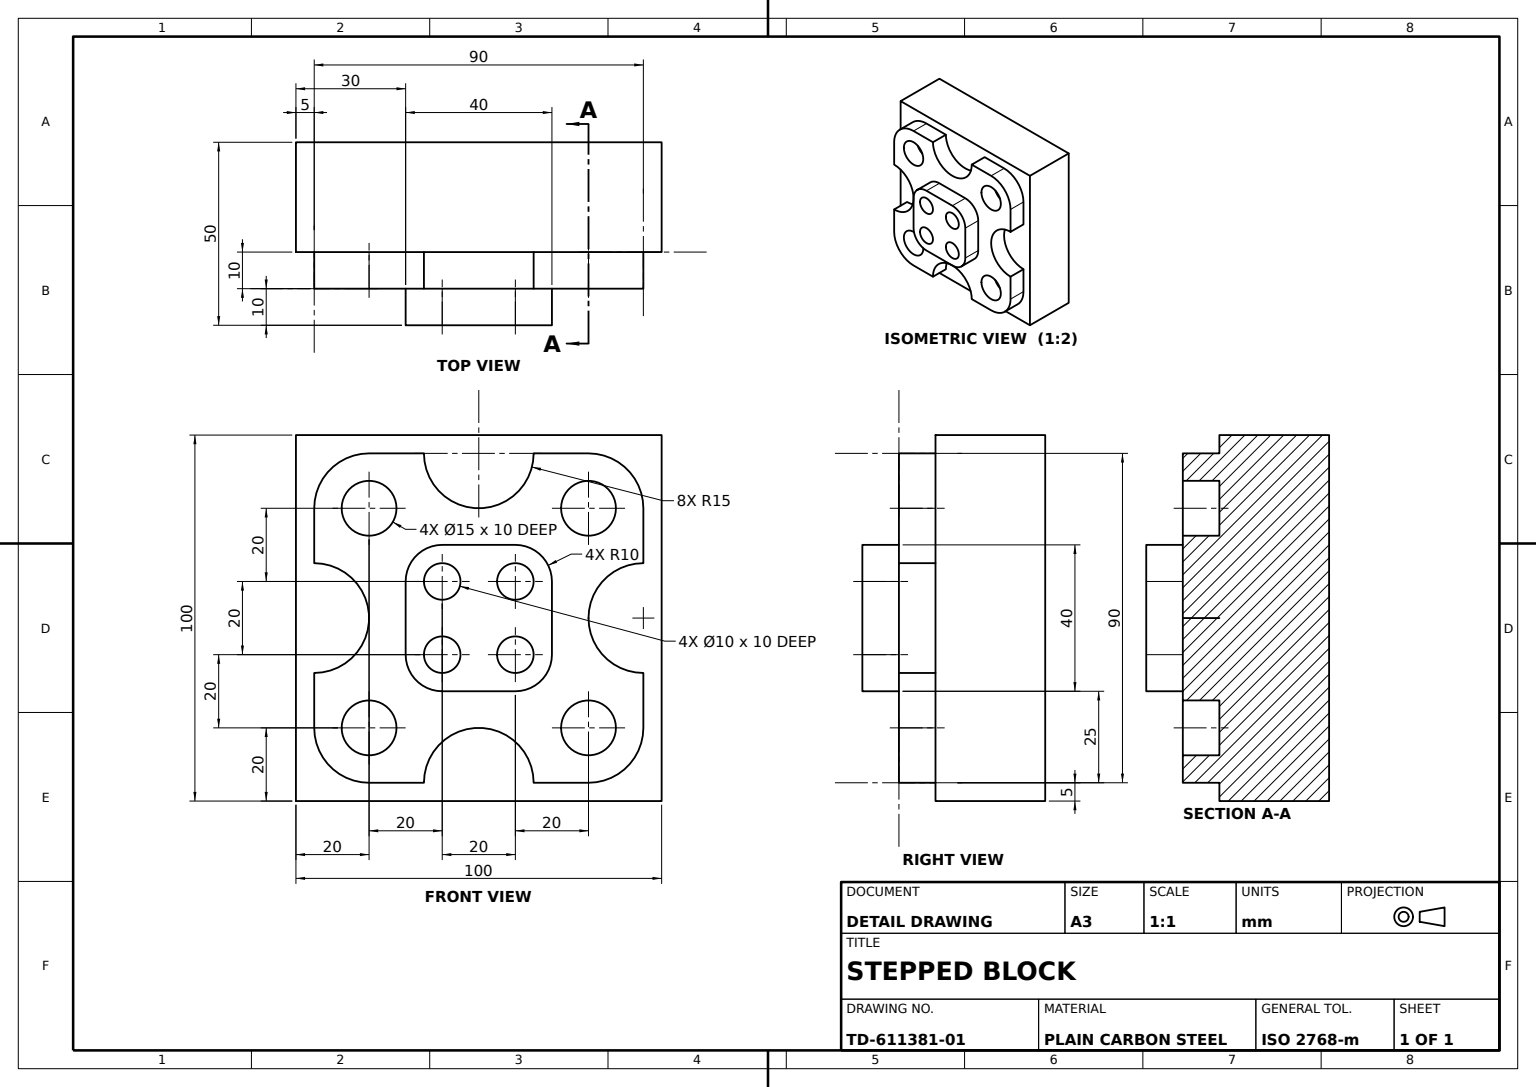
ISO-10303-21;
HEADER;
FILE_DESCRIPTION((''),'2;1');
FILE_NAME('','',(''),(''),'','','');
FILE_SCHEMA(('AUTOMOTIVE_DESIGN'));
ENDSEC;
DATA;
#1=APPLICATION_CONTEXT('');
#2=PRODUCT_CONTEXT('',#1,'mechanical');
#3=PRODUCT('','','',(#2));
#4=PRODUCT_DEFINITION_FORMATION('','',#3);
#5=PRODUCT_DEFINITION_CONTEXT('',#1,'design');
#6=PRODUCT_DEFINITION('','',#4,#5);
#7=PRODUCT_DEFINITION_SHAPE('','',#6);
#8=(LENGTH_UNIT()NAMED_UNIT(*)SI_UNIT(.MILLI.,.METRE.));
#9=(NAMED_UNIT(*)PLANE_ANGLE_UNIT()SI_UNIT($,.RADIAN.));
#10=(NAMED_UNIT(*)SI_UNIT($,.STERADIAN.)SOLID_ANGLE_UNIT());
#11=UNCERTAINTY_MEASURE_WITH_UNIT(LENGTH_MEASURE(1.E-05),#8,'distance_accuracy_value','');
#12=(GEOMETRIC_REPRESENTATION_CONTEXT(3)GLOBAL_UNCERTAINTY_ASSIGNED_CONTEXT((#11))GLOBAL_UNIT_ASSIGNED_CONTEXT((#8,#9,#10))REPRESENTATION_CONTEXT('',''));
#13=CARTESIAN_POINT('',(-22.5,-35.,-15.));
#14=VERTEX_POINT('',#13);
#15=CARTESIAN_POINT('',(-22.5,-35.,-25.));
#16=VERTEX_POINT('',#15);
#17=DIRECTION('',(0.,0.,-1.));
#18=VECTOR('',#17,1000.);
#19=LINE('',#13,#18);
#20=EDGE_CURVE('',#14,#16,#19,.T.);
#21=ORIENTED_EDGE('',*,*,#20,.T.);
#22=CARTESIAN_POINT('',(-37.5,-35.,-25.));
#23=VERTEX_POINT('',#22);
#24=CARTESIAN_POINT('',(-30.,-35.,-25.));
#25=DIRECTION('',(-1.,0.,0.));
#26=AXIS2_PLACEMENT_3D('',#24,#17,#25);
#27=CIRCLE('',#26,7.5);
#28=EDGE_CURVE('',#16,#23,#27,.T.);
#29=ORIENTED_EDGE('',*,*,#28,.T.);
#30=CARTESIAN_POINT('',(-37.5,-35.,-15.));
#31=VERTEX_POINT('',#30);
#32=LINE('',#30,#18);
#33=EDGE_CURVE('',#31,#23,#32,.T.);
#34=ORIENTED_EDGE('',*,*,#33,.F.);
#35=CARTESIAN_POINT('',(-30.,-35.,-15.));
#36=AXIS2_PLACEMENT_3D('',#35,#17,#25);
#37=CIRCLE('',#36,7.5);
#38=EDGE_CURVE('',#14,#31,#37,.T.);
#39=ORIENTED_EDGE('',*,*,#38,.F.);
#40=EDGE_LOOP('',(#21,#29,#34,#39));
#41=FACE_OUTER_BOUND('',#40,.T.);
#42=CYLINDRICAL_SURFACE('',#36,7.5);
#43=ADVANCED_FACE('',(#41),#42,.F.);
#44=CARTESIAN_POINT('',(15.,5.,-25.));
#45=VERTEX_POINT('',#44);
#46=CARTESIAN_POINT('',(5.,5.,-25.));
#47=VERTEX_POINT('',#46);
#48=CARTESIAN_POINT('',(10.,5.,-25.));
#49=AXIS2_PLACEMENT_3D('',#48,#17,#25);
#50=CIRCLE('',#49,5.);
#51=EDGE_CURVE('',#45,#47,#50,.T.);
#52=ORIENTED_EDGE('',*,*,#51,.F.);
#53=CARTESIAN_POINT('',(15.,5.,-35.));
#54=VERTEX_POINT('',#53);
#55=LINE('',#44,#18);
#56=EDGE_CURVE('',#45,#54,#55,.T.);
#57=ORIENTED_EDGE('',*,*,#56,.T.);
#58=CARTESIAN_POINT('',(5.,5.,-35.));
#59=VERTEX_POINT('',#58);
#60=CARTESIAN_POINT('',(10.,5.,-35.));
#61=AXIS2_PLACEMENT_3D('',#60,#17,#25);
#62=CIRCLE('',#61,5.);
#63=EDGE_CURVE('',#54,#59,#62,.T.);
#64=ORIENTED_EDGE('',*,*,#63,.T.);
#65=LINE('',#46,#18);
#66=EDGE_CURVE('',#47,#59,#65,.T.);
#67=ORIENTED_EDGE('',*,*,#66,.F.);
#68=EDGE_LOOP('',(#52,#57,#64,#67));
#69=FACE_OUTER_BOUND('',#68,.T.);
#70=CYLINDRICAL_SURFACE('',#49,5.);
#71=ADVANCED_FACE('',(#69),#70,.F.);
#72=CARTESIAN_POINT('',(-15.,5.,-35.));
#73=VERTEX_POINT('',#72);
#74=CARTESIAN_POINT('',(-5.,5.,-35.));
#75=VERTEX_POINT('',#74);
#76=CARTESIAN_POINT('',(-10.,5.,-35.));
#77=AXIS2_PLACEMENT_3D('',#76,#17,#25);
#78=CIRCLE('',#77,5.);
#79=EDGE_CURVE('',#73,#75,#78,.T.);
#80=ORIENTED_EDGE('',*,*,#79,.F.);
#81=EDGE_CURVE('',#75,#73,#78,.T.);
#82=ORIENTED_EDGE('',*,*,#81,.F.);
#83=EDGE_LOOP('',(#80,#82));
#84=FACE_BOUND('',#83,.T.);
#85=CARTESIAN_POINT('',(5.,-15.,-35.));
#86=VERTEX_POINT('',#85);
#87=CARTESIAN_POINT('',(15.,-15.,-35.));
#88=VERTEX_POINT('',#87);
#89=CARTESIAN_POINT('',(10.,-15.,-35.));
#90=AXIS2_PLACEMENT_3D('',#89,#17,#25);
#91=CIRCLE('',#90,5.);
#92=EDGE_CURVE('',#86,#88,#91,.T.);
#93=ORIENTED_EDGE('',*,*,#92,.F.);
#94=EDGE_CURVE('',#88,#86,#91,.T.);
#95=ORIENTED_EDGE('',*,*,#94,.F.);
#96=EDGE_LOOP('',(#93,#95));
#97=FACE_BOUND('',#96,.T.);
#98=CARTESIAN_POINT('',(-5.,-15.,-35.));
#99=VERTEX_POINT('',#98);
#100=CARTESIAN_POINT('',(-15.,-15.,-35.));
#101=VERTEX_POINT('',#100);
#102=CARTESIAN_POINT('',(-10.,-15.,-35.));
#103=AXIS2_PLACEMENT_3D('',#102,#17,#25);
#104=CIRCLE('',#103,5.);
#105=EDGE_CURVE('',#99,#101,#104,.T.);
#106=ORIENTED_EDGE('',*,*,#105,.F.);
#107=EDGE_CURVE('',#101,#99,#104,.T.);
#108=ORIENTED_EDGE('',*,*,#107,.F.);
#109=EDGE_LOOP('',(#106,#108));
#110=FACE_BOUND('',#109,.T.);
#111=CARTESIAN_POINT('',(10.,15.,-35.));
#112=VERTEX_POINT('',#111);
#113=CARTESIAN_POINT('',(20.,5.,-35.));
#114=VERTEX_POINT('',#113);
#115=CIRCLE('',#61,10.);
#116=EDGE_CURVE('',#112,#114,#115,.T.);
#117=ORIENTED_EDGE('',*,*,#116,.T.);
#118=CARTESIAN_POINT('',(20.,-15.,-35.));
#119=VERTEX_POINT('',#118);
#120=CARTESIAN_POINT('',(20.,15.,-35.));
#121=DIRECTION('',(0.,-1.,0.));
#122=VECTOR('',#121,1000.);
#123=LINE('',#120,#122);
#124=EDGE_CURVE('',#114,#119,#123,.T.);
#125=ORIENTED_EDGE('',*,*,#124,.T.);
#126=CARTESIAN_POINT('',(10.,-25.,-35.));
#127=VERTEX_POINT('',#126);
#128=CIRCLE('',#90,10.);
#129=EDGE_CURVE('',#119,#127,#128,.T.);
#130=ORIENTED_EDGE('',*,*,#129,.T.);
#131=CARTESIAN_POINT('',(-10.,-25.,-35.));
#132=VERTEX_POINT('',#131);
#133=CARTESIAN_POINT('',(20.,-25.,-35.));
#134=VECTOR('',#25,1000.);
#135=LINE('',#133,#134);
#136=EDGE_CURVE('',#127,#132,#135,.T.);
#137=ORIENTED_EDGE('',*,*,#136,.T.);
#138=CARTESIAN_POINT('',(-20.,-15.,-35.));
#139=VERTEX_POINT('',#138);
#140=CIRCLE('',#103,10.);
#141=EDGE_CURVE('',#132,#139,#140,.T.);
#142=ORIENTED_EDGE('',*,*,#141,.T.);
#143=CARTESIAN_POINT('',(-20.,5.,-35.));
#144=VERTEX_POINT('',#143);
#145=CARTESIAN_POINT('',(-20.,-25.,-35.));
#146=DIRECTION('',(0.,1.,0.));
#147=VECTOR('',#146,1000.);
#148=LINE('',#145,#147);
#149=EDGE_CURVE('',#139,#144,#148,.T.);
#150=ORIENTED_EDGE('',*,*,#149,.T.);
#151=CARTESIAN_POINT('',(-10.,15.,-35.));
#152=VERTEX_POINT('',#151);
#153=CIRCLE('',#77,10.);
#154=EDGE_CURVE('',#144,#152,#153,.T.);
#155=ORIENTED_EDGE('',*,*,#154,.T.);
#156=CARTESIAN_POINT('',(-20.,15.,-35.));
#157=DIRECTION('',(1.,0.,0.));
#158=VECTOR('',#157,1000.);
#159=LINE('',#156,#158);
#160=EDGE_CURVE('',#152,#112,#159,.T.);
#161=ORIENTED_EDGE('',*,*,#160,.T.);
#162=EDGE_LOOP('',(#117,#125,#130,#137,#142,#150,#155,#161));
#163=FACE_OUTER_BOUND('',#162,.T.);
#164=EDGE_CURVE('',#59,#54,#62,.T.);
#165=ORIENTED_EDGE('',*,*,#164,.F.);
#166=ORIENTED_EDGE('',*,*,#63,.F.);
#167=EDGE_LOOP('',(#165,#166));
#168=FACE_BOUND('',#167,.T.);
#169=CARTESIAN_POINT('',(0.,0.,-35.));
#170=AXIS2_PLACEMENT_3D('',#169,#17,#25);
#171=PLANE('',#170);
#172=ADVANCED_FACE('',(#84,#97,#110,#163,#168),#171,.T.);
#173=CARTESIAN_POINT('',(22.5,25.,-15.));
#174=VERTEX_POINT('',#173);
#175=CARTESIAN_POINT('',(22.5,25.,-25.));
#176=VERTEX_POINT('',#175);
#177=LINE('',#173,#18);
#178=EDGE_CURVE('',#174,#176,#177,.T.);
#179=ORIENTED_EDGE('',*,*,#178,.T.);
#180=CARTESIAN_POINT('',(37.5,25.,-25.));
#181=VERTEX_POINT('',#180);
#182=CARTESIAN_POINT('',(30.,25.,-25.));
#183=AXIS2_PLACEMENT_3D('',#182,#17,#25);
#184=CIRCLE('',#183,7.5);
#185=EDGE_CURVE('',#176,#181,#184,.T.);
#186=ORIENTED_EDGE('',*,*,#185,.T.);
#187=CARTESIAN_POINT('',(37.5,25.,-15.));
#188=VERTEX_POINT('',#187);
#189=LINE('',#187,#18);
#190=EDGE_CURVE('',#188,#181,#189,.T.);
#191=ORIENTED_EDGE('',*,*,#190,.F.);
#192=CARTESIAN_POINT('',(30.,25.,-15.));
#193=AXIS2_PLACEMENT_3D('',#192,#17,#25);
#194=CIRCLE('',#193,7.5);
#195=EDGE_CURVE('',#174,#188,#194,.T.);
#196=ORIENTED_EDGE('',*,*,#195,.F.);
#197=EDGE_LOOP('',(#179,#186,#191,#196));
#198=FACE_OUTER_BOUND('',#197,.T.);
#199=CYLINDRICAL_SURFACE('',#193,7.5);
#200=ADVANCED_FACE('',(#198),#199,.F.);
#201=CARTESIAN_POINT('',(15.,-15.,-25.));
#202=VERTEX_POINT('',#201);
#203=CARTESIAN_POINT('',(5.,-15.,-25.));
#204=VERTEX_POINT('',#203);
#205=CARTESIAN_POINT('',(10.,-15.,-25.));
#206=AXIS2_PLACEMENT_3D('',#205,#17,#25);
#207=CIRCLE('',#206,5.);
#208=EDGE_CURVE('',#202,#204,#207,.T.);
#209=ORIENTED_EDGE('',*,*,#208,.F.);
#210=LINE('',#201,#18);
#211=EDGE_CURVE('',#202,#88,#210,.T.);
#212=ORIENTED_EDGE('',*,*,#211,.T.);
#213=ORIENTED_EDGE('',*,*,#94,.T.);
#214=LINE('',#203,#18);
#215=EDGE_CURVE('',#204,#86,#214,.T.);
#216=ORIENTED_EDGE('',*,*,#215,.F.);
#217=EDGE_LOOP('',(#209,#212,#213,#216));
#218=FACE_OUTER_BOUND('',#217,.T.);
#219=CYLINDRICAL_SURFACE('',#206,5.);
#220=ADVANCED_FACE('',(#218),#219,.F.);
#221=CARTESIAN_POINT('',(50.,45.,-15.));
#222=VERTEX_POINT('',#221);
#223=CARTESIAN_POINT('',(-50.,45.,-15.));
#224=VERTEX_POINT('',#223);
#225=LINE('',#221,#134);
#226=EDGE_CURVE('',#222,#224,#225,.T.);
#227=ORIENTED_EDGE('',*,*,#226,.T.);
#228=CARTESIAN_POINT('',(-50.,45.,15.));
#229=VERTEX_POINT('',#228);
#230=LINE('',#228,#18);
#231=EDGE_CURVE('',#229,#224,#230,.T.);
#232=ORIENTED_EDGE('',*,*,#231,.F.);
#233=CARTESIAN_POINT('',(50.,45.,15.));
#234=VERTEX_POINT('',#233);
#235=LINE('',#233,#134);
#236=EDGE_CURVE('',#234,#229,#235,.T.);
#237=ORIENTED_EDGE('',*,*,#236,.F.);
#238=LINE('',#233,#18);
#239=EDGE_CURVE('',#234,#222,#238,.T.);
#240=ORIENTED_EDGE('',*,*,#239,.T.);
#241=EDGE_LOOP('',(#227,#232,#237,#240));
#242=FACE_OUTER_BOUND('',#241,.T.);
#243=AXIS2_PLACEMENT_3D('',#233,#121,#157);
#244=PLANE('',#243);
#245=ADVANCED_FACE('',(#242),#244,.F.);
#246=CARTESIAN_POINT('',(-10.,-25.,-25.));
#247=VERTEX_POINT('',#246);
#248=LINE('',#131,#18);
#249=EDGE_CURVE('',#247,#132,#248,.T.);
#250=ORIENTED_EDGE('',*,*,#249,.F.);
#251=CARTESIAN_POINT('',(-20.,-15.,-25.));
#252=VERTEX_POINT('',#251);
#253=CARTESIAN_POINT('',(-10.,-15.,-25.));
#254=DIRECTION('',(0.,0.,1.));
#255=AXIS2_PLACEMENT_3D('',#253,#254,#25);
#256=CIRCLE('',#255,10.);
#257=EDGE_CURVE('',#252,#247,#256,.T.);
#258=ORIENTED_EDGE('',*,*,#257,.F.);
#259=VECTOR('',#254,1000.);
#260=LINE('',#138,#259);
#261=EDGE_CURVE('',#139,#252,#260,.T.);
#262=ORIENTED_EDGE('',*,*,#261,.F.);
#263=ORIENTED_EDGE('',*,*,#141,.F.);
#264=EDGE_LOOP('',(#250,#258,#262,#263));
#265=FACE_OUTER_BOUND('',#264,.T.);
#266=AXIS2_PLACEMENT_3D('',#102,#254,#157);
#267=CYLINDRICAL_SURFACE('',#266,10.);
#268=ADVANCED_FACE('',(#265),#267,.T.);
#269=CARTESIAN_POINT('',(-5.,5.,-25.));
#270=VERTEX_POINT('',#269);
#271=LINE('',#269,#18);
#272=EDGE_CURVE('',#270,#75,#271,.T.);
#273=ORIENTED_EDGE('',*,*,#272,.T.);
#274=ORIENTED_EDGE('',*,*,#81,.T.);
#275=CARTESIAN_POINT('',(-15.,5.,-25.));
#276=VERTEX_POINT('',#275);
#277=LINE('',#275,#18);
#278=EDGE_CURVE('',#276,#73,#277,.T.);
#279=ORIENTED_EDGE('',*,*,#278,.F.);
#280=CARTESIAN_POINT('',(-10.,5.,-25.));
#281=AXIS2_PLACEMENT_3D('',#280,#17,#25);
#282=CIRCLE('',#281,5.);
#283=EDGE_CURVE('',#270,#276,#282,.T.);
#284=ORIENTED_EDGE('',*,*,#283,.F.);
#285=EDGE_LOOP('',(#273,#274,#279,#284));
#286=FACE_OUTER_BOUND('',#285,.T.);
#287=CYLINDRICAL_SURFACE('',#281,5.);
#288=ADVANCED_FACE('',(#286),#287,.F.);
#289=CARTESIAN_POINT('',(-45.,-35.,-15.));
#290=VERTEX_POINT('',#289);
#291=CARTESIAN_POINT('',(-30.,-50.,-15.));
#292=VERTEX_POINT('',#291);
#293=AXIS2_PLACEMENT_3D('',#35,#254,#157);
#294=CIRCLE('',#293,15.);
#295=EDGE_CURVE('',#290,#292,#294,.T.);
#296=ORIENTED_EDGE('',*,*,#295,.T.);
#297=CARTESIAN_POINT('',(-15.,-50.,-15.));
#298=VERTEX_POINT('',#297);
#299=CARTESIAN_POINT('',(-45.,-50.,-15.));
#300=LINE('',#299,#134);
#301=EDGE_CURVE('',#298,#292,#300,.T.);
#302=ORIENTED_EDGE('',*,*,#301,.F.);
#303=CARTESIAN_POINT('',(15.,-50.,-15.));
#304=VERTEX_POINT('',#303);
#305=CARTESIAN_POINT('',(0.,-50.,-15.));
#306=AXIS2_PLACEMENT_3D('',#305,#254,#25);
#307=CIRCLE('',#306,15.);
#308=EDGE_CURVE('',#304,#298,#307,.T.);
#309=ORIENTED_EDGE('',*,*,#308,.F.);
#310=CARTESIAN_POINT('',(30.,-50.,-15.));
#311=VERTEX_POINT('',#310);
#312=LINE('',#303,#134);
#313=EDGE_CURVE('',#311,#304,#312,.T.);
#314=ORIENTED_EDGE('',*,*,#313,.F.);
#315=CARTESIAN_POINT('',(45.,-35.,-15.));
#316=VERTEX_POINT('',#315);
#317=CARTESIAN_POINT('',(30.,-35.,-15.));
#318=AXIS2_PLACEMENT_3D('',#317,#254,#157);
#319=CIRCLE('',#318,15.);
#320=EDGE_CURVE('',#311,#316,#319,.T.);
#321=ORIENTED_EDGE('',*,*,#320,.T.);
#322=CARTESIAN_POINT('',(45.,-20.,-15.));
#323=VERTEX_POINT('',#322);
#324=CARTESIAN_POINT('',(45.,-50.,-15.));
#325=LINE('',#324,#122);
#326=EDGE_CURVE('',#323,#316,#325,.T.);
#327=ORIENTED_EDGE('',*,*,#326,.F.);
#328=CARTESIAN_POINT('',(45.,10.,-15.));
#329=VERTEX_POINT('',#328);
#330=CARTESIAN_POINT('',(45.,-5.,-15.));
#331=AXIS2_PLACEMENT_3D('',#330,#254,#25);
#332=CIRCLE('',#331,15.);
#333=EDGE_CURVE('',#329,#323,#332,.T.);
#334=ORIENTED_EDGE('',*,*,#333,.F.);
#335=CARTESIAN_POINT('',(45.,25.,-15.));
#336=VERTEX_POINT('',#335);
#337=LINE('',#328,#122);
#338=EDGE_CURVE('',#336,#329,#337,.T.);
#339=ORIENTED_EDGE('',*,*,#338,.F.);
#340=CARTESIAN_POINT('',(30.,40.,-15.));
#341=VERTEX_POINT('',#340);
#342=AXIS2_PLACEMENT_3D('',#192,#254,#157);
#343=CIRCLE('',#342,15.);
#344=EDGE_CURVE('',#336,#341,#343,.T.);
#345=ORIENTED_EDGE('',*,*,#344,.T.);
#346=CARTESIAN_POINT('',(15.,40.,-15.));
#347=VERTEX_POINT('',#346);
#348=CARTESIAN_POINT('',(45.,40.,-15.));
#349=LINE('',#348,#158);
#350=EDGE_CURVE('',#347,#341,#349,.T.);
#351=ORIENTED_EDGE('',*,*,#350,.F.);
#352=CARTESIAN_POINT('',(-15.,40.,-15.));
#353=VERTEX_POINT('',#352);
#354=CARTESIAN_POINT('',(0.,40.,-15.));
#355=AXIS2_PLACEMENT_3D('',#354,#254,#25);
#356=CIRCLE('',#355,15.);
#357=EDGE_CURVE('',#353,#347,#356,.T.);
#358=ORIENTED_EDGE('',*,*,#357,.F.);
#359=CARTESIAN_POINT('',(-30.,40.,-15.));
#360=VERTEX_POINT('',#359);
#361=LINE('',#352,#158);
#362=EDGE_CURVE('',#360,#353,#361,.T.);
#363=ORIENTED_EDGE('',*,*,#362,.F.);
#364=CARTESIAN_POINT('',(-45.,25.,-15.));
#365=VERTEX_POINT('',#364);
#366=CARTESIAN_POINT('',(-30.,25.,-15.));
#367=AXIS2_PLACEMENT_3D('',#366,#254,#157);
#368=CIRCLE('',#367,15.);
#369=EDGE_CURVE('',#360,#365,#368,.T.);
#370=ORIENTED_EDGE('',*,*,#369,.T.);
#371=CARTESIAN_POINT('',(-45.,10.,-15.));
#372=VERTEX_POINT('',#371);
#373=CARTESIAN_POINT('',(-45.,40.,-15.));
#374=LINE('',#373,#147);
#375=EDGE_CURVE('',#372,#365,#374,.T.);
#376=ORIENTED_EDGE('',*,*,#375,.F.);
#377=CARTESIAN_POINT('',(-30.,-5.,-15.));
#378=VERTEX_POINT('',#377);
#379=CARTESIAN_POINT('',(-45.,-5.,-15.));
#380=AXIS2_PLACEMENT_3D('',#379,#254,#25);
#381=CIRCLE('',#380,15.);
#382=EDGE_CURVE('',#378,#372,#381,.T.);
#383=ORIENTED_EDGE('',*,*,#382,.F.);
#384=CARTESIAN_POINT('',(-45.,-20.,-15.));
#385=VERTEX_POINT('',#384);
#386=EDGE_CURVE('',#385,#378,#381,.T.);
#387=ORIENTED_EDGE('',*,*,#386,.F.);
#388=LINE('',#384,#147);
#389=EDGE_CURVE('',#290,#385,#388,.T.);
#390=ORIENTED_EDGE('',*,*,#389,.F.);
#391=EDGE_LOOP('',(#296,#302,#309,#314,#321,#327,#334,#339,#345,#351,#358,#363,#370,#376,#383,#387,#390));
#392=FACE_BOUND('',#391,.T.);
#393=CARTESIAN_POINT('',(50.,-55.,-15.));
#394=VERTEX_POINT('',#393);
#395=CARTESIAN_POINT('',(50.,0.,-15.));
#396=LINE('',#395,#147);
#397=EDGE_CURVE('',#394,#222,#396,.T.);
#398=ORIENTED_EDGE('',*,*,#397,.F.);
#399=CARTESIAN_POINT('',(-50.,-55.,-15.));
#400=VERTEX_POINT('',#399);
#401=LINE('',#399,#158);
#402=EDGE_CURVE('',#400,#394,#401,.T.);
#403=ORIENTED_EDGE('',*,*,#402,.F.);
#404=LINE('',#223,#122);
#405=EDGE_CURVE('',#224,#400,#404,.T.);
#406=ORIENTED_EDGE('',*,*,#405,.F.);
#407=ORIENTED_EDGE('',*,*,#226,.F.);
#408=EDGE_LOOP('',(#398,#403,#406,#407));
#409=FACE_OUTER_BOUND('',#408,.T.);
#410=CARTESIAN_POINT('',(0.,0.,-15.));
#411=AXIS2_PLACEMENT_3D('',#410,#254,#157);
#412=PLANE('',#411);
#413=ADVANCED_FACE('',(#392,#409),#412,.F.);
#414=ORIENTED_EDGE('',*,*,#129,.F.);
#415=CARTESIAN_POINT('',(20.,-15.,-25.));
#416=VERTEX_POINT('',#415);
#417=LINE('',#118,#18);
#418=EDGE_CURVE('',#416,#119,#417,.T.);
#419=ORIENTED_EDGE('',*,*,#418,.F.);
#420=CARTESIAN_POINT('',(10.,-25.,-25.));
#421=VERTEX_POINT('',#420);
#422=AXIS2_PLACEMENT_3D('',#205,#254,#25);
#423=CIRCLE('',#422,10.);
#424=EDGE_CURVE('',#421,#416,#423,.T.);
#425=ORIENTED_EDGE('',*,*,#424,.F.);
#426=LINE('',#126,#259);
#427=EDGE_CURVE('',#127,#421,#426,.T.);
#428=ORIENTED_EDGE('',*,*,#427,.F.);
#429=EDGE_LOOP('',(#414,#419,#425,#428));
#430=FACE_OUTER_BOUND('',#429,.T.);
#431=AXIS2_PLACEMENT_3D('',#89,#254,#157);
#432=CYLINDRICAL_SURFACE('',#431,10.);
#433=ADVANCED_FACE('',(#430),#432,.T.);
#434=CARTESIAN_POINT('',(45.,-20.,-25.));
#435=VERTEX_POINT('',#434);
#436=LINE('',#434,#259);
#437=EDGE_CURVE('',#435,#323,#436,.T.);
#438=ORIENTED_EDGE('',*,*,#437,.T.);
#439=ORIENTED_EDGE('',*,*,#326,.T.);
#440=CARTESIAN_POINT('',(45.,-35.,-25.));
#441=VERTEX_POINT('',#440);
#442=LINE('',#440,#18);
#443=EDGE_CURVE('',#316,#441,#442,.T.);
#444=ORIENTED_EDGE('',*,*,#443,.T.);
#445=CARTESIAN_POINT('',(45.,-50.,-25.));
#446=LINE('',#445,#122);
#447=EDGE_CURVE('',#435,#441,#446,.T.);
#448=ORIENTED_EDGE('',*,*,#447,.F.);
#449=EDGE_LOOP('',(#438,#439,#444,#448));
#450=FACE_OUTER_BOUND('',#449,.T.);
#451=AXIS2_PLACEMENT_3D('',#445,#25,#254);
#452=PLANE('',#451);
#453=ADVANCED_FACE('',(#450),#452,.F.);
#454=CARTESIAN_POINT('',(30.,-50.,-25.));
#455=VERTEX_POINT('',#454);
#456=LINE('',#454,#259);
#457=EDGE_CURVE('',#455,#311,#456,.T.);
#458=ORIENTED_EDGE('',*,*,#457,.T.);
#459=ORIENTED_EDGE('',*,*,#313,.T.);
#460=CARTESIAN_POINT('',(15.,-50.,-25.));
#461=VERTEX_POINT('',#460);
#462=LINE('',#460,#259);
#463=EDGE_CURVE('',#461,#304,#462,.T.);
#464=ORIENTED_EDGE('',*,*,#463,.F.);
#465=LINE('',#460,#134);
#466=EDGE_CURVE('',#455,#461,#465,.T.);
#467=ORIENTED_EDGE('',*,*,#466,.F.);
#468=EDGE_LOOP('',(#458,#459,#464,#467));
#469=FACE_OUTER_BOUND('',#468,.T.);
#470=AXIS2_PLACEMENT_3D('',#460,#146,#25);
#471=PLANE('',#470);
#472=ADVANCED_FACE('',(#469),#471,.F.);
#473=ORIENTED_EDGE('',*,*,#283,.T.);
#474=EDGE_CURVE('',#276,#270,#282,.T.);
#475=ORIENTED_EDGE('',*,*,#474,.T.);
#476=EDGE_LOOP('',(#473,#475));
#477=FACE_OUTER_BOUND('',#476,.T.);
#478=PLANE('',#281);
#479=ADVANCED_FACE('',(#477),#478,.T.);
#480=CARTESIAN_POINT('',(20.,5.,-25.));
#481=VERTEX_POINT('',#480);
#482=LINE('',#113,#259);
#483=EDGE_CURVE('',#114,#481,#482,.T.);
#484=ORIENTED_EDGE('',*,*,#483,.T.);
#485=CARTESIAN_POINT('',(20.,15.,-25.));
#486=LINE('',#485,#122);
#487=EDGE_CURVE('',#481,#416,#486,.T.);
#488=ORIENTED_EDGE('',*,*,#487,.T.);
#489=ORIENTED_EDGE('',*,*,#418,.T.);
#490=ORIENTED_EDGE('',*,*,#124,.F.);
#491=EDGE_LOOP('',(#484,#488,#489,#490));
#492=FACE_OUTER_BOUND('',#491,.T.);
#493=AXIS2_PLACEMENT_3D('',#120,#25,#121);
#494=PLANE('',#493);
#495=ADVANCED_FACE('',(#492),#494,.F.);
#496=CARTESIAN_POINT('',(10.,15.,-25.));
#497=VERTEX_POINT('',#496);
#498=AXIS2_PLACEMENT_3D('',#48,#254,#25);
#499=CIRCLE('',#498,10.);
#500=EDGE_CURVE('',#481,#497,#499,.T.);
#501=ORIENTED_EDGE('',*,*,#500,.F.);
#502=ORIENTED_EDGE('',*,*,#483,.F.);
#503=ORIENTED_EDGE('',*,*,#116,.F.);
#504=LINE('',#111,#18);
#505=EDGE_CURVE('',#497,#112,#504,.T.);
#506=ORIENTED_EDGE('',*,*,#505,.F.);
#507=EDGE_LOOP('',(#501,#502,#503,#506));
#508=FACE_OUTER_BOUND('',#507,.T.);
#509=AXIS2_PLACEMENT_3D('',#60,#254,#157);
#510=CYLINDRICAL_SURFACE('',#509,10.);
#511=ADVANCED_FACE('',(#508),#510,.T.);
#512=ORIENTED_EDGE('',*,*,#457,.F.);
#513=CARTESIAN_POINT('',(30.,-35.,-25.));
#514=AXIS2_PLACEMENT_3D('',#513,#17,#25);
#515=CIRCLE('',#514,15.);
#516=EDGE_CURVE('',#441,#455,#515,.T.);
#517=ORIENTED_EDGE('',*,*,#516,.F.);
#518=ORIENTED_EDGE('',*,*,#443,.F.);
#519=ORIENTED_EDGE('',*,*,#320,.F.);
#520=EDGE_LOOP('',(#512,#517,#518,#519));
#521=FACE_OUTER_BOUND('',#520,.T.);
#522=AXIS2_PLACEMENT_3D('',#513,#254,#157);
#523=CYLINDRICAL_SURFACE('',#522,15.);
#524=ADVANCED_FACE('',(#521),#523,.T.);
#525=ORIENTED_EDGE('',*,*,#231,.T.);
#526=ORIENTED_EDGE('',*,*,#405,.T.);
#527=CARTESIAN_POINT('',(-50.,-55.,15.));
#528=VERTEX_POINT('',#527);
#529=LINE('',#527,#18);
#530=EDGE_CURVE('',#528,#400,#529,.T.);
#531=ORIENTED_EDGE('',*,*,#530,.F.);
#532=LINE('',#228,#122);
#533=EDGE_CURVE('',#229,#528,#532,.T.);
#534=ORIENTED_EDGE('',*,*,#533,.F.);
#535=EDGE_LOOP('',(#525,#526,#531,#534));
#536=FACE_OUTER_BOUND('',#535,.T.);
#537=AXIS2_PLACEMENT_3D('',#228,#157,#146);
#538=PLANE('',#537);
#539=ADVANCED_FACE('',(#536),#538,.F.);
#540=ORIENTED_EDGE('',*,*,#530,.T.);
#541=ORIENTED_EDGE('',*,*,#402,.T.);
#542=CARTESIAN_POINT('',(50.,-55.,15.));
#543=VERTEX_POINT('',#542);
#544=LINE('',#542,#18);
#545=EDGE_CURVE('',#543,#394,#544,.T.);
#546=ORIENTED_EDGE('',*,*,#545,.F.);
#547=LINE('',#527,#158);
#548=EDGE_CURVE('',#528,#543,#547,.T.);
#549=ORIENTED_EDGE('',*,*,#548,.F.);
#550=EDGE_LOOP('',(#540,#541,#546,#549));
#551=FACE_OUTER_BOUND('',#550,.T.);
#552=AXIS2_PLACEMENT_3D('',#527,#146,#254);
#553=PLANE('',#552);
#554=ADVANCED_FACE('',(#551),#553,.F.);
#555=CARTESIAN_POINT('',(-45.,25.,-25.));
#556=VERTEX_POINT('',#555);
#557=LINE('',#555,#18);
#558=EDGE_CURVE('',#365,#556,#557,.T.);
#559=ORIENTED_EDGE('',*,*,#558,.T.);
#560=CARTESIAN_POINT('',(-45.,10.,-25.));
#561=VERTEX_POINT('',#560);
#562=CARTESIAN_POINT('',(-45.,40.,-25.));
#563=LINE('',#562,#147);
#564=EDGE_CURVE('',#561,#556,#563,.T.);
#565=ORIENTED_EDGE('',*,*,#564,.F.);
#566=LINE('',#560,#259);
#567=EDGE_CURVE('',#561,#372,#566,.T.);
#568=ORIENTED_EDGE('',*,*,#567,.T.);
#569=ORIENTED_EDGE('',*,*,#375,.T.);
#570=EDGE_LOOP('',(#559,#565,#568,#569));
#571=FACE_OUTER_BOUND('',#570,.T.);
#572=AXIS2_PLACEMENT_3D('',#562,#157,#146);
#573=PLANE('',#572);
#574=ADVANCED_FACE('',(#571),#573,.F.);
#575=ORIENTED_EDGE('',*,*,#149,.F.);
#576=ORIENTED_EDGE('',*,*,#261,.T.);
#577=CARTESIAN_POINT('',(-20.,5.,-25.));
#578=VERTEX_POINT('',#577);
#579=CARTESIAN_POINT('',(-20.,-25.,-25.));
#580=LINE('',#579,#147);
#581=EDGE_CURVE('',#252,#578,#580,.T.);
#582=ORIENTED_EDGE('',*,*,#581,.T.);
#583=LINE('',#143,#18);
#584=EDGE_CURVE('',#578,#144,#583,.T.);
#585=ORIENTED_EDGE('',*,*,#584,.T.);
#586=EDGE_LOOP('',(#575,#576,#582,#585));
#587=FACE_OUTER_BOUND('',#586,.T.);
#588=AXIS2_PLACEMENT_3D('',#145,#157,#17);
#589=PLANE('',#588);
#590=ADVANCED_FACE('',(#587),#589,.F.);
#591=CARTESIAN_POINT('',(30.,40.,-25.));
#592=VERTEX_POINT('',#591);
#593=LINE('',#591,#18);
#594=EDGE_CURVE('',#341,#592,#593,.T.);
#595=ORIENTED_EDGE('',*,*,#594,.T.);
#596=CARTESIAN_POINT('',(15.,40.,-25.));
#597=VERTEX_POINT('',#596);
#598=CARTESIAN_POINT('',(45.,40.,-25.));
#599=LINE('',#598,#158);
#600=EDGE_CURVE('',#597,#592,#599,.T.);
#601=ORIENTED_EDGE('',*,*,#600,.F.);
#602=LINE('',#596,#259);
#603=EDGE_CURVE('',#597,#347,#602,.T.);
#604=ORIENTED_EDGE('',*,*,#603,.T.);
#605=ORIENTED_EDGE('',*,*,#350,.T.);
#606=EDGE_LOOP('',(#595,#601,#604,#605));
#607=FACE_OUTER_BOUND('',#606,.T.);
#608=AXIS2_PLACEMENT_3D('',#598,#121,#17);
#609=PLANE('',#608);
#610=ADVANCED_FACE('',(#607),#609,.F.);
#611=ORIENTED_EDGE('',*,*,#272,.F.);
#612=ORIENTED_EDGE('',*,*,#474,.F.);
#613=ORIENTED_EDGE('',*,*,#278,.T.);
#614=ORIENTED_EDGE('',*,*,#79,.T.);
#615=EDGE_LOOP('',(#611,#612,#613,#614));
#616=FACE_OUTER_BOUND('',#615,.T.);
#617=ADVANCED_FACE('',(#616),#287,.F.);
#618=ORIENTED_EDGE('',*,*,#239,.F.);
#619=LINE('',#542,#147);
#620=EDGE_CURVE('',#543,#234,#619,.T.);
#621=ORIENTED_EDGE('',*,*,#620,.F.);
#622=ORIENTED_EDGE('',*,*,#545,.T.);
#623=ORIENTED_EDGE('',*,*,#397,.T.);
#624=EDGE_LOOP('',(#618,#621,#622,#623));
#625=FACE_OUTER_BOUND('',#624,.T.);
#626=CARTESIAN_POINT('',(50.,0.,15.));
#627=AXIS2_PLACEMENT_3D('',#626,#25,#254);
#628=PLANE('',#627);
#629=ADVANCED_FACE('',(#625),#628,.F.);
#630=EDGE_CURVE('',#23,#16,#27,.T.);
#631=ORIENTED_EDGE('',*,*,#630,.F.);
#632=ORIENTED_EDGE('',*,*,#28,.F.);
#633=EDGE_LOOP('',(#631,#632));
#634=FACE_BOUND('',#633,.T.);
#635=CARTESIAN_POINT('',(22.5,-35.,-25.));
#636=VERTEX_POINT('',#635);
#637=CARTESIAN_POINT('',(37.5,-35.,-25.));
#638=VERTEX_POINT('',#637);
#639=CIRCLE('',#514,7.5);
#640=EDGE_CURVE('',#636,#638,#639,.T.);
#641=ORIENTED_EDGE('',*,*,#640,.F.);
#642=EDGE_CURVE('',#638,#636,#639,.T.);
#643=ORIENTED_EDGE('',*,*,#642,.F.);
#644=EDGE_LOOP('',(#641,#643));
#645=FACE_BOUND('',#644,.T.);
#646=CARTESIAN_POINT('',(-22.5,25.,-25.));
#647=VERTEX_POINT('',#646);
#648=CARTESIAN_POINT('',(-37.5,25.,-25.));
#649=VERTEX_POINT('',#648);
#650=CARTESIAN_POINT('',(-30.,25.,-25.));
#651=AXIS2_PLACEMENT_3D('',#650,#17,#25);
#652=CIRCLE('',#651,7.5);
#653=EDGE_CURVE('',#647,#649,#652,.T.);
#654=ORIENTED_EDGE('',*,*,#653,.F.);
#655=EDGE_CURVE('',#649,#647,#652,.T.);
#656=ORIENTED_EDGE('',*,*,#655,.F.);
#657=EDGE_LOOP('',(#654,#656));
#658=FACE_BOUND('',#657,.T.);
#659=ORIENTED_EDGE('',*,*,#185,.F.);
#660=EDGE_CURVE('',#181,#176,#184,.T.);
#661=ORIENTED_EDGE('',*,*,#660,.F.);
#662=EDGE_LOOP('',(#659,#661));
#663=FACE_BOUND('',#662,.T.);
#664=ORIENTED_EDGE('',*,*,#564,.T.);
#665=CARTESIAN_POINT('',(-30.,40.,-25.));
#666=VERTEX_POINT('',#665);
#667=CIRCLE('',#651,15.);
#668=EDGE_CURVE('',#556,#666,#667,.T.);
#669=ORIENTED_EDGE('',*,*,#668,.T.);
#670=CARTESIAN_POINT('',(-15.,40.,-25.));
#671=VERTEX_POINT('',#670);
#672=LINE('',#670,#158);
#673=EDGE_CURVE('',#666,#671,#672,.T.);
#674=ORIENTED_EDGE('',*,*,#673,.T.);
#675=CARTESIAN_POINT('',(0.,40.,-25.));
#676=AXIS2_PLACEMENT_3D('',#675,#254,#25);
#677=CIRCLE('',#676,15.);
#678=EDGE_CURVE('',#671,#597,#677,.T.);
#679=ORIENTED_EDGE('',*,*,#678,.T.);
#680=ORIENTED_EDGE('',*,*,#600,.T.);
#681=CARTESIAN_POINT('',(45.,25.,-25.));
#682=VERTEX_POINT('',#681);
#683=CIRCLE('',#183,15.);
#684=EDGE_CURVE('',#592,#682,#683,.T.);
#685=ORIENTED_EDGE('',*,*,#684,.T.);
#686=CARTESIAN_POINT('',(45.,10.,-25.));
#687=VERTEX_POINT('',#686);
#688=LINE('',#686,#122);
#689=EDGE_CURVE('',#682,#687,#688,.T.);
#690=ORIENTED_EDGE('',*,*,#689,.T.);
#691=CARTESIAN_POINT('',(45.,-5.,-25.));
#692=AXIS2_PLACEMENT_3D('',#691,#254,#25);
#693=CIRCLE('',#692,15.);
#694=EDGE_CURVE('',#687,#435,#693,.T.);
#695=ORIENTED_EDGE('',*,*,#694,.T.);
#696=ORIENTED_EDGE('',*,*,#447,.T.);
#697=ORIENTED_EDGE('',*,*,#516,.T.);
#698=ORIENTED_EDGE('',*,*,#466,.T.);
#699=CARTESIAN_POINT('',(-15.,-50.,-25.));
#700=VERTEX_POINT('',#699);
#701=CARTESIAN_POINT('',(0.,-50.,-25.));
#702=AXIS2_PLACEMENT_3D('',#701,#254,#25);
#703=CIRCLE('',#702,15.);
#704=EDGE_CURVE('',#461,#700,#703,.T.);
#705=ORIENTED_EDGE('',*,*,#704,.T.);
#706=CARTESIAN_POINT('',(-30.,-50.,-25.));
#707=VERTEX_POINT('',#706);
#708=CARTESIAN_POINT('',(-45.,-50.,-25.));
#709=LINE('',#708,#134);
#710=EDGE_CURVE('',#700,#707,#709,.T.);
#711=ORIENTED_EDGE('',*,*,#710,.T.);
#712=CARTESIAN_POINT('',(-45.,-35.,-25.));
#713=VERTEX_POINT('',#712);
#714=CIRCLE('',#26,15.);
#715=EDGE_CURVE('',#707,#713,#714,.T.);
#716=ORIENTED_EDGE('',*,*,#715,.T.);
#717=CARTESIAN_POINT('',(-45.,-20.,-25.));
#718=VERTEX_POINT('',#717);
#719=LINE('',#717,#147);
#720=EDGE_CURVE('',#713,#718,#719,.T.);
#721=ORIENTED_EDGE('',*,*,#720,.T.);
#722=CARTESIAN_POINT('',(-30.,-5.,-25.));
#723=VERTEX_POINT('',#722);
#724=CARTESIAN_POINT('',(-45.,-5.,-25.));
#725=AXIS2_PLACEMENT_3D('',#724,#254,#25);
#726=CIRCLE('',#725,15.);
#727=EDGE_CURVE('',#718,#723,#726,.T.);
#728=ORIENTED_EDGE('',*,*,#727,.T.);
#729=EDGE_CURVE('',#723,#561,#726,.T.);
#730=ORIENTED_EDGE('',*,*,#729,.T.);
#731=EDGE_LOOP('',(#664,#669,#674,#679,#680,#685,#690,#695,#696,#697,#698,#705,#711,#716,#721,#728,#730));
#732=FACE_OUTER_BOUND('',#731,.T.);
#733=ORIENTED_EDGE('',*,*,#581,.F.);
#734=ORIENTED_EDGE('',*,*,#257,.T.);
#735=CARTESIAN_POINT('',(0.,-25.,-25.));
#736=LINE('',#735,#134);
#737=EDGE_CURVE('',#421,#247,#736,.T.);
#738=ORIENTED_EDGE('',*,*,#737,.F.);
#739=ORIENTED_EDGE('',*,*,#424,.T.);
#740=ORIENTED_EDGE('',*,*,#487,.F.);
#741=ORIENTED_EDGE('',*,*,#500,.T.);
#742=CARTESIAN_POINT('',(-10.,15.,-25.));
#743=VERTEX_POINT('',#742);
#744=CARTESIAN_POINT('',(-20.,15.,-25.));
#745=LINE('',#744,#158);
#746=EDGE_CURVE('',#743,#497,#745,.T.);
#747=ORIENTED_EDGE('',*,*,#746,.F.);
#748=AXIS2_PLACEMENT_3D('',#280,#254,#25);
#749=CIRCLE('',#748,10.);
#750=EDGE_CURVE('',#743,#578,#749,.T.);
#751=ORIENTED_EDGE('',*,*,#750,.T.);
#752=EDGE_LOOP('',(#733,#734,#738,#739,#740,#741,#747,#751));
#753=FACE_BOUND('',#752,.T.);
#754=AXIS2_PLACEMENT_3D('',#701,#17,#25);
#755=PLANE('',#754);
#756=ADVANCED_FACE('',(#634,#645,#658,#663,#732,#753),#755,.T.);
#757=ORIENTED_EDGE('',*,*,#215,.T.);
#758=ORIENTED_EDGE('',*,*,#92,.T.);
#759=ORIENTED_EDGE('',*,*,#211,.F.);
#760=EDGE_CURVE('',#204,#202,#207,.T.);
#761=ORIENTED_EDGE('',*,*,#760,.F.);
#762=EDGE_LOOP('',(#757,#758,#759,#761));
#763=FACE_OUTER_BOUND('',#762,.T.);
#764=ADVANCED_FACE('',(#763),#219,.F.);
#765=ORIENTED_EDGE('',*,*,#338,.T.);
#766=LINE('',#686,#259);
#767=EDGE_CURVE('',#687,#329,#766,.T.);
#768=ORIENTED_EDGE('',*,*,#767,.F.);
#769=ORIENTED_EDGE('',*,*,#689,.F.);
#770=LINE('',#681,#259);
#771=EDGE_CURVE('',#682,#336,#770,.T.);
#772=ORIENTED_EDGE('',*,*,#771,.T.);
#773=EDGE_LOOP('',(#765,#768,#769,#772));
#774=FACE_OUTER_BOUND('',#773,.T.);
#775=AXIS2_PLACEMENT_3D('',#686,#25,#254);
#776=PLANE('',#775);
#777=ADVANCED_FACE('',(#774),#776,.F.);
#778=CARTESIAN_POINT('',(22.5,-35.,-15.));
#779=VERTEX_POINT('',#778);
#780=CARTESIAN_POINT('',(37.5,-35.,-15.));
#781=VERTEX_POINT('',#780);
#782=AXIS2_PLACEMENT_3D('',#317,#17,#25);
#783=CIRCLE('',#782,7.5);
#784=EDGE_CURVE('',#779,#781,#783,.T.);
#785=ORIENTED_EDGE('',*,*,#784,.T.);
#786=EDGE_CURVE('',#781,#779,#783,.T.);
#787=ORIENTED_EDGE('',*,*,#786,.T.);
#788=EDGE_LOOP('',(#785,#787));
#789=FACE_OUTER_BOUND('',#788,.T.);
#790=PLANE('',#782);
#791=ADVANCED_FACE('',(#789),#790,.T.);
#792=ORIENTED_EDGE('',*,*,#694,.F.);
#793=ORIENTED_EDGE('',*,*,#767,.T.);
#794=ORIENTED_EDGE('',*,*,#333,.T.);
#795=ORIENTED_EDGE('',*,*,#437,.F.);
#796=EDGE_LOOP('',(#792,#793,#794,#795));
#797=FACE_OUTER_BOUND('',#796,.T.);
#798=AXIS2_PLACEMENT_3D('',#691,#254,#157);
#799=CYLINDRICAL_SURFACE('',#798,15.);
#800=ADVANCED_FACE('',(#797),#799,.F.);
#801=ORIENTED_EDGE('',*,*,#673,.F.);
#802=LINE('',#665,#259);
#803=EDGE_CURVE('',#666,#360,#802,.T.);
#804=ORIENTED_EDGE('',*,*,#803,.T.);
#805=ORIENTED_EDGE('',*,*,#362,.T.);
#806=LINE('',#670,#259);
#807=EDGE_CURVE('',#671,#353,#806,.T.);
#808=ORIENTED_EDGE('',*,*,#807,.F.);
#809=EDGE_LOOP('',(#801,#804,#805,#808));
#810=FACE_OUTER_BOUND('',#809,.T.);
#811=AXIS2_PLACEMENT_3D('',#670,#121,#17);
#812=PLANE('',#811);
#813=ADVANCED_FACE('',(#810),#812,.F.);
#814=LINE('',#722,#259);
#815=EDGE_CURVE('',#723,#378,#814,.T.);
#816=ORIENTED_EDGE('',*,*,#815,.T.);
#817=ORIENTED_EDGE('',*,*,#382,.T.);
#818=ORIENTED_EDGE('',*,*,#567,.F.);
#819=ORIENTED_EDGE('',*,*,#729,.F.);
#820=EDGE_LOOP('',(#816,#817,#818,#819));
#821=FACE_OUTER_BOUND('',#820,.T.);
#822=AXIS2_PLACEMENT_3D('',#724,#254,#157);
#823=CYLINDRICAL_SURFACE('',#822,15.);
#824=ADVANCED_FACE('',(#821),#823,.F.);
#825=ORIENTED_EDGE('',*,*,#369,.F.);
#826=ORIENTED_EDGE('',*,*,#803,.F.);
#827=ORIENTED_EDGE('',*,*,#668,.F.);
#828=ORIENTED_EDGE('',*,*,#558,.F.);
#829=EDGE_LOOP('',(#825,#826,#827,#828));
#830=FACE_OUTER_BOUND('',#829,.T.);
#831=AXIS2_PLACEMENT_3D('',#650,#254,#157);
#832=CYLINDRICAL_SURFACE('',#831,15.);
#833=ADVANCED_FACE('',(#830),#832,.T.);
#834=ORIENTED_EDGE('',*,*,#750,.F.);
#835=LINE('',#151,#259);
#836=EDGE_CURVE('',#152,#743,#835,.T.);
#837=ORIENTED_EDGE('',*,*,#836,.F.);
#838=ORIENTED_EDGE('',*,*,#154,.F.);
#839=ORIENTED_EDGE('',*,*,#584,.F.);
#840=EDGE_LOOP('',(#834,#837,#838,#839));
#841=FACE_OUTER_BOUND('',#840,.T.);
#842=AXIS2_PLACEMENT_3D('',#76,#254,#157);
#843=CYLINDRICAL_SURFACE('',#842,10.);
#844=ADVANCED_FACE('',(#841),#843,.T.);
#845=CARTESIAN_POINT('',(-15.,-15.,-25.));
#846=VERTEX_POINT('',#845);
#847=LINE('',#845,#18);
#848=EDGE_CURVE('',#846,#101,#847,.T.);
#849=ORIENTED_EDGE('',*,*,#848,.F.);
#850=CARTESIAN_POINT('',(-5.,-15.,-25.));
#851=VERTEX_POINT('',#850);
#852=AXIS2_PLACEMENT_3D('',#253,#17,#25);
#853=CIRCLE('',#852,5.);
#854=EDGE_CURVE('',#851,#846,#853,.T.);
#855=ORIENTED_EDGE('',*,*,#854,.F.);
#856=LINE('',#850,#18);
#857=EDGE_CURVE('',#851,#99,#856,.T.);
#858=ORIENTED_EDGE('',*,*,#857,.T.);
#859=ORIENTED_EDGE('',*,*,#105,.T.);
#860=EDGE_LOOP('',(#849,#855,#858,#859));
#861=FACE_OUTER_BOUND('',#860,.T.);
#862=CYLINDRICAL_SURFACE('',#852,5.);
#863=ADVANCED_FACE('',(#861),#862,.F.);
#864=ORIENTED_EDGE('',*,*,#807,.T.);
#865=ORIENTED_EDGE('',*,*,#357,.T.);
#866=ORIENTED_EDGE('',*,*,#603,.F.);
#867=ORIENTED_EDGE('',*,*,#678,.F.);
#868=EDGE_LOOP('',(#864,#865,#866,#867));
#869=FACE_OUTER_BOUND('',#868,.T.);
#870=AXIS2_PLACEMENT_3D('',#675,#254,#157);
#871=CYLINDRICAL_SURFACE('',#870,15.);
#872=ADVANCED_FACE('',(#869),#871,.F.);
#873=ORIENTED_EDGE('',*,*,#594,.F.);
#874=ORIENTED_EDGE('',*,*,#344,.F.);
#875=ORIENTED_EDGE('',*,*,#771,.F.);
#876=ORIENTED_EDGE('',*,*,#684,.F.);
#877=EDGE_LOOP('',(#873,#874,#875,#876));
#878=FACE_OUTER_BOUND('',#877,.T.);
#879=AXIS2_PLACEMENT_3D('',#182,#254,#157);
#880=CYLINDRICAL_SURFACE('',#879,15.);
#881=ADVANCED_FACE('',(#878),#880,.T.);
#882=LINE('',#780,#18);
#883=EDGE_CURVE('',#781,#638,#882,.T.);
#884=ORIENTED_EDGE('',*,*,#883,.T.);
#885=ORIENTED_EDGE('',*,*,#642,.T.);
#886=LINE('',#778,#18);
#887=EDGE_CURVE('',#779,#636,#886,.T.);
#888=ORIENTED_EDGE('',*,*,#887,.F.);
#889=ORIENTED_EDGE('',*,*,#786,.F.);
#890=EDGE_LOOP('',(#884,#885,#888,#889));
#891=FACE_OUTER_BOUND('',#890,.T.);
#892=CYLINDRICAL_SURFACE('',#782,7.5);
#893=ADVANCED_FACE('',(#891),#892,.F.);
#894=ORIENTED_EDGE('',*,*,#20,.F.);
#895=EDGE_CURVE('',#31,#14,#37,.T.);
#896=ORIENTED_EDGE('',*,*,#895,.F.);
#897=ORIENTED_EDGE('',*,*,#33,.T.);
#898=ORIENTED_EDGE('',*,*,#630,.T.);
#899=EDGE_LOOP('',(#894,#896,#897,#898));
#900=FACE_OUTER_BOUND('',#899,.T.);
#901=ADVANCED_FACE('',(#900),#42,.F.);
#902=LINE('',#706,#18);
#903=EDGE_CURVE('',#292,#707,#902,.T.);
#904=ORIENTED_EDGE('',*,*,#903,.T.);
#905=ORIENTED_EDGE('',*,*,#710,.F.);
#906=LINE('',#699,#259);
#907=EDGE_CURVE('',#700,#298,#906,.T.);
#908=ORIENTED_EDGE('',*,*,#907,.T.);
#909=ORIENTED_EDGE('',*,*,#301,.T.);
#910=EDGE_LOOP('',(#904,#905,#908,#909));
#911=FACE_OUTER_BOUND('',#910,.T.);
#912=AXIS2_PLACEMENT_3D('',#708,#146,#254);
#913=PLANE('',#912);
#914=ADVANCED_FACE('',(#911),#913,.F.);
#915=ORIENTED_EDGE('',*,*,#854,.T.);
#916=EDGE_CURVE('',#846,#851,#853,.T.);
#917=ORIENTED_EDGE('',*,*,#916,.T.);
#918=EDGE_LOOP('',(#915,#917));
#919=FACE_OUTER_BOUND('',#918,.T.);
#920=PLANE('',#852);
#921=ADVANCED_FACE('',(#919),#920,.T.);
#922=ORIENTED_EDGE('',*,*,#815,.F.);
#923=ORIENTED_EDGE('',*,*,#727,.F.);
#924=LINE('',#717,#259);
#925=EDGE_CURVE('',#718,#385,#924,.T.);
#926=ORIENTED_EDGE('',*,*,#925,.T.);
#927=ORIENTED_EDGE('',*,*,#386,.T.);
#928=EDGE_LOOP('',(#922,#923,#926,#927));
#929=FACE_OUTER_BOUND('',#928,.T.);
#930=ADVANCED_FACE('',(#929),#823,.F.);
#931=CARTESIAN_POINT('',(-37.5,25.,-15.));
#932=VERTEX_POINT('',#931);
#933=LINE('',#931,#18);
#934=EDGE_CURVE('',#932,#649,#933,.T.);
#935=ORIENTED_EDGE('',*,*,#934,.T.);
#936=ORIENTED_EDGE('',*,*,#655,.T.);
#937=CARTESIAN_POINT('',(-22.5,25.,-15.));
#938=VERTEX_POINT('',#937);
#939=LINE('',#937,#18);
#940=EDGE_CURVE('',#938,#647,#939,.T.);
#941=ORIENTED_EDGE('',*,*,#940,.F.);
#942=AXIS2_PLACEMENT_3D('',#366,#17,#25);
#943=CIRCLE('',#942,7.5);
#944=EDGE_CURVE('',#932,#938,#943,.T.);
#945=ORIENTED_EDGE('',*,*,#944,.F.);
#946=EDGE_LOOP('',(#935,#936,#941,#945));
#947=FACE_OUTER_BOUND('',#946,.T.);
#948=CYLINDRICAL_SURFACE('',#942,7.5);
#949=ADVANCED_FACE('',(#947),#948,.F.);
#950=ORIENTED_EDGE('',*,*,#704,.F.);
#951=ORIENTED_EDGE('',*,*,#463,.T.);
#952=ORIENTED_EDGE('',*,*,#308,.T.);
#953=ORIENTED_EDGE('',*,*,#907,.F.);
#954=EDGE_LOOP('',(#950,#951,#952,#953));
#955=FACE_OUTER_BOUND('',#954,.T.);
#956=AXIS2_PLACEMENT_3D('',#701,#254,#157);
#957=CYLINDRICAL_SURFACE('',#956,15.);
#958=ADVANCED_FACE('',(#955),#957,.F.);
#959=ORIENTED_EDGE('',*,*,#903,.F.);
#960=ORIENTED_EDGE('',*,*,#295,.F.);
#961=LINE('',#712,#259);
#962=EDGE_CURVE('',#713,#290,#961,.T.);
#963=ORIENTED_EDGE('',*,*,#962,.F.);
#964=ORIENTED_EDGE('',*,*,#715,.F.);
#965=EDGE_LOOP('',(#959,#960,#963,#964));
#966=FACE_OUTER_BOUND('',#965,.T.);
#967=AXIS2_PLACEMENT_3D('',#24,#254,#157);
#968=CYLINDRICAL_SURFACE('',#967,15.);
#969=ADVANCED_FACE('',(#966),#968,.T.);
#970=ORIENTED_EDGE('',*,*,#178,.F.);
#971=EDGE_CURVE('',#188,#174,#194,.T.);
#972=ORIENTED_EDGE('',*,*,#971,.F.);
#973=ORIENTED_EDGE('',*,*,#190,.T.);
#974=ORIENTED_EDGE('',*,*,#660,.T.);
#975=EDGE_LOOP('',(#970,#972,#973,#974));
#976=FACE_OUTER_BOUND('',#975,.T.);
#977=ADVANCED_FACE('',(#976),#199,.F.);
#978=ORIENTED_EDGE('',*,*,#934,.F.);
#979=EDGE_CURVE('',#938,#932,#943,.T.);
#980=ORIENTED_EDGE('',*,*,#979,.F.);
#981=ORIENTED_EDGE('',*,*,#940,.T.);
#982=ORIENTED_EDGE('',*,*,#653,.T.);
#983=EDGE_LOOP('',(#978,#980,#981,#982));
#984=FACE_OUTER_BOUND('',#983,.T.);
#985=ADVANCED_FACE('',(#984),#948,.F.);
#986=ORIENTED_EDGE('',*,*,#857,.F.);
#987=ORIENTED_EDGE('',*,*,#916,.F.);
#988=ORIENTED_EDGE('',*,*,#848,.T.);
#989=ORIENTED_EDGE('',*,*,#107,.T.);
#990=EDGE_LOOP('',(#986,#987,#988,#989));
#991=FACE_OUTER_BOUND('',#990,.T.);
#992=ADVANCED_FACE('',(#991),#862,.F.);
#993=ORIENTED_EDGE('',*,*,#720,.F.);
#994=ORIENTED_EDGE('',*,*,#962,.T.);
#995=ORIENTED_EDGE('',*,*,#389,.T.);
#996=ORIENTED_EDGE('',*,*,#925,.F.);
#997=EDGE_LOOP('',(#993,#994,#995,#996));
#998=FACE_OUTER_BOUND('',#997,.T.);
#999=AXIS2_PLACEMENT_3D('',#717,#157,#146);
#1000=PLANE('',#999);
#1001=ADVANCED_FACE('',(#998),#1000,.F.);
#1002=ORIENTED_EDGE('',*,*,#160,.F.);
#1003=ORIENTED_EDGE('',*,*,#836,.T.);
#1004=ORIENTED_EDGE('',*,*,#746,.T.);
#1005=ORIENTED_EDGE('',*,*,#505,.T.);
#1006=EDGE_LOOP('',(#1002,#1003,#1004,#1005));
#1007=FACE_OUTER_BOUND('',#1006,.T.);
#1008=AXIS2_PLACEMENT_3D('',#156,#121,#157);
#1009=PLANE('',#1008);
#1010=ADVANCED_FACE('',(#1007),#1009,.F.);
#1011=ORIENTED_EDGE('',*,*,#427,.T.);
#1012=ORIENTED_EDGE('',*,*,#737,.T.);
#1013=ORIENTED_EDGE('',*,*,#249,.T.);
#1014=ORIENTED_EDGE('',*,*,#136,.F.);
#1015=EDGE_LOOP('',(#1011,#1012,#1013,#1014));
#1016=FACE_OUTER_BOUND('',#1015,.T.);
#1017=CARTESIAN_POINT('',(0.,-25.,-35.));
#1018=AXIS2_PLACEMENT_3D('',#1017,#146,#254);
#1019=PLANE('',#1018);
#1020=ADVANCED_FACE('',(#1016),#1019,.F.);
#1021=ORIENTED_EDGE('',*,*,#979,.T.);
#1022=ORIENTED_EDGE('',*,*,#944,.T.);
#1023=EDGE_LOOP('',(#1021,#1022));
#1024=FACE_OUTER_BOUND('',#1023,.T.);
#1025=PLANE('',#942);
#1026=ADVANCED_FACE('',(#1024),#1025,.T.);
#1027=ORIENTED_EDGE('',*,*,#38,.T.);
#1028=ORIENTED_EDGE('',*,*,#895,.T.);
#1029=EDGE_LOOP('',(#1027,#1028));
#1030=FACE_OUTER_BOUND('',#1029,.T.);
#1031=PLANE('',#36);
#1032=ADVANCED_FACE('',(#1030),#1031,.T.);
#1033=ORIENTED_EDGE('',*,*,#66,.T.);
#1034=ORIENTED_EDGE('',*,*,#164,.T.);
#1035=ORIENTED_EDGE('',*,*,#56,.F.);
#1036=EDGE_CURVE('',#47,#45,#50,.T.);
#1037=ORIENTED_EDGE('',*,*,#1036,.F.);
#1038=EDGE_LOOP('',(#1033,#1034,#1035,#1037));
#1039=FACE_OUTER_BOUND('',#1038,.T.);
#1040=ADVANCED_FACE('',(#1039),#70,.F.);
#1041=ORIENTED_EDGE('',*,*,#533,.T.);
#1042=ORIENTED_EDGE('',*,*,#548,.T.);
#1043=ORIENTED_EDGE('',*,*,#620,.T.);
#1044=ORIENTED_EDGE('',*,*,#236,.T.);
#1045=EDGE_LOOP('',(#1041,#1042,#1043,#1044));
#1046=FACE_OUTER_BOUND('',#1045,.T.);
#1047=CARTESIAN_POINT('',(0.,0.,15.));
#1048=AXIS2_PLACEMENT_3D('',#1047,#254,#157);
#1049=PLANE('',#1048);
#1050=ADVANCED_FACE('',(#1046),#1049,.T.);
#1051=ORIENTED_EDGE('',*,*,#760,.T.);
#1052=ORIENTED_EDGE('',*,*,#208,.T.);
#1053=EDGE_LOOP('',(#1051,#1052));
#1054=FACE_OUTER_BOUND('',#1053,.T.);
#1055=PLANE('',#206);
#1056=ADVANCED_FACE('',(#1054),#1055,.T.);
#1057=ORIENTED_EDGE('',*,*,#971,.T.);
#1058=ORIENTED_EDGE('',*,*,#195,.T.);
#1059=EDGE_LOOP('',(#1057,#1058));
#1060=FACE_OUTER_BOUND('',#1059,.T.);
#1061=PLANE('',#193);
#1062=ADVANCED_FACE('',(#1060),#1061,.T.);
#1063=ORIENTED_EDGE('',*,*,#887,.T.);
#1064=ORIENTED_EDGE('',*,*,#640,.T.);
#1065=ORIENTED_EDGE('',*,*,#883,.F.);
#1066=ORIENTED_EDGE('',*,*,#784,.F.);
#1067=EDGE_LOOP('',(#1063,#1064,#1065,#1066));
#1068=FACE_OUTER_BOUND('',#1067,.T.);
#1069=ADVANCED_FACE('',(#1068),#892,.F.);
#1070=ORIENTED_EDGE('',*,*,#51,.T.);
#1071=ORIENTED_EDGE('',*,*,#1036,.T.);
#1072=EDGE_LOOP('',(#1070,#1071));
#1073=FACE_OUTER_BOUND('',#1072,.T.);
#1074=PLANE('',#49);
#1075=ADVANCED_FACE('',(#1073),#1074,.T.);
#1076=CLOSED_SHELL('',(#43,#71,#172,#200,#220,#245,#268,#288,#413,#433,#453,#472,#479,#495,#511,#524,#539,#554,#574,#590,#610,#617,#629,#756,#764,#777,#791,#800,#813,#824,#833,#844,#863,#872,#881,#893,#901,#914,#921,#930,#949,#958,#969,#977,#985,#992,#1001,#1010,#1020,#1026,#1032,#1040,#1050,#1056,#1062,#1069,#1075));
#1077=MANIFOLD_SOLID_BREP('',#1076);
#1078=ADVANCED_BREP_SHAPE_REPRESENTATION('',(#1077),#12);
#1079=SHAPE_DEFINITION_REPRESENTATION(#7,#1078);
ENDSEC;
END-ISO-10303-21;
